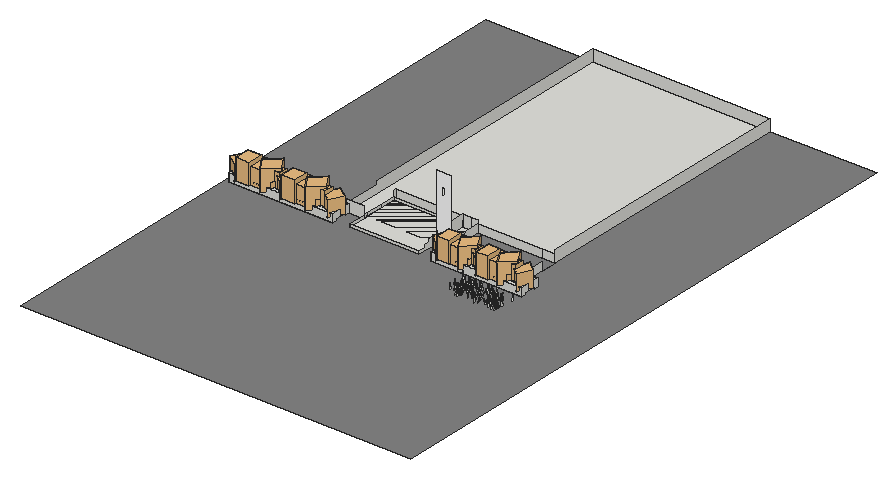
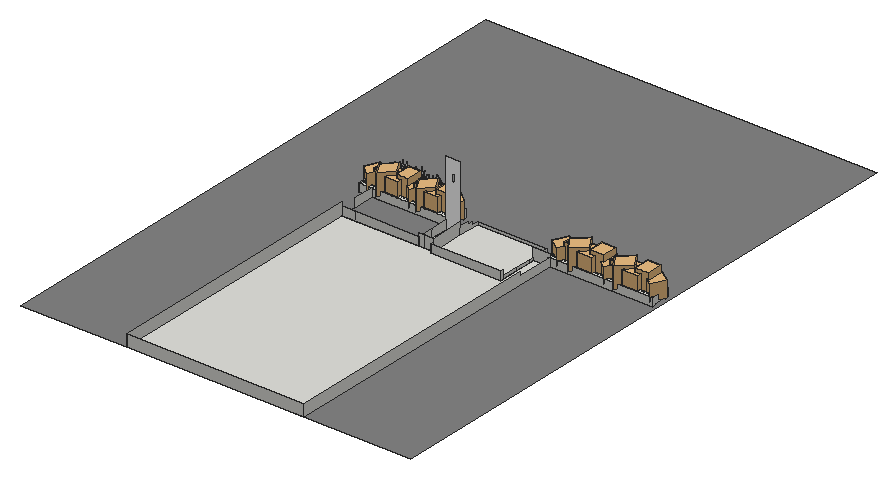
# SketchUp Ruby script. Lengths in inches.
U = 1.inch
M = Sketchup.active_model
def pt(a) = Geom::Point3d.new(a.map { |v| v * U })
def face(e, loops, mat)
  f = e.add_face(loops[0].map { |a| pt(a) })
  loops[1..].each { |l| e.add_face(l.map { |a| pt(a) }).erase! }
  f.material = f.back_material = mat if mat
  f
end
# faces: each face lists its corners as indices into pts; further lists are holes
def faces(e, pts, list, mat = nil) = list.each { |f| face(e, (f[0].is_a?(Array) ? f : [f]).map { |l| l.map { |i| pts[i] } }, mat) }
# xy, xz, yz: faces in a plane at the given z, y or x. An outline is a flat list of corners, or four numbers for a rectangle; further outlines are holes
def ring(l) = l.size == 4 ? [[l[0], l[1]], [l[2], l[1]], [l[2], l[3]], [l[0], l[3]]] : l.each_slice(2).to_a
def flat(e, list, mat, &to3) = list.each { |f| face(e, (f[0].is_a?(Array) ? f : [f]).map { |l| ring(l).map { |u, v| to3.(u, v) } }, mat) }
def xy(e, z, list, mat = nil) = flat(e, list, mat) { |x, y| [x, y, z] }
def xz(e, y, list, mat = nil) = flat(e, list, mat) { |x, z| [x, y, z] }
def yz(e, x, list, mat = nil) = flat(e, list, mat) { |y, z| [x, y, z] }
def lines(e, pts, list) = list.each { |a, b| e.add_line(pt(pts[a]), pt(pts[b])) }
# prism: a flat outline (further loops are holes) pulled along v
def prism(e, loops, v, mat = nil)
  f = face(e, loops, mat); d = Geom::Vector3d.new(v.map { |x| x * U })
  f.pushpull(f.normal.samedirection?(d) ? d.length : -d.length)
end
def box(e, o, s, mat = nil) = prism(e, [[o, [o[0] + s[0], o[1], o[2]], [o[0] + s[0], o[1] + s[1], o[2]], [o[0], o[1] + s[1], o[2]]]], [0, 0, s[2]], mat)
def at(x, y, z, deg = 0) = Geom::Transformation.translation(pt([x, y, z])) * Geom::Transformation.rotation(ORIGIN, Z_AXIS, deg.degrees)
def axes(o, x, y, z) = Geom::Transformation.new([*x, 0, *y, 0, *z, 0, *pt(o).to_a, 1])
def part(name) = M.definitions.add(name)
# library, detail: a bought-in or finely detailed component or shape, given as its bounding box
def library(name, o, s) = part(name).tap { |d| box(d.entities, o, s) }
def detail(e, o, s) = box(e.add_group.entities, o, s)
def put(e, d, t, mat = nil) = e.add_instance(d, t).tap { |i| i.material = mat if mat }
def group(e, t, mat = nil) = e.add_group.tap { |g| g.transformation = t; g.material = mat if mat }.entities
root = M.entities
M.materials.add("Material__1").color = [95, 70, 46]
M.materials.add("[Color M00]").color = [255, 255, 255]
M.materials.add("[Tile Grey]").color = [132, 132, 132]
c1 = part("fur_instance\#9")
p = [[0.8125,0,1.79],[0.67,-0.02,1.48],[0,-0.11,0],[0,0.11,0]]
faces(c1.entities,p,[[0,1,2,3]])
c2 = library("Areca palm plant",[0,0,0],[49.1,36.6,54.46])
c3 = library("Group\#74",[-84.69,-90.07,-0.36],[176.51,175.13,171.4])
c4 = library("Group20\#1",[-20.81,-17.08,3.79],[39.86,39.43,37.51])
c5 = library("Group\#130",[-7.34,-1.2,0],[38.67,35.81,49.04])
c6 = library("Group38\#2",[14.01,28.44,-23.43],[18.58,18.32,38.89])
c7 = part("Group\#69")
put(c7.entities,c2,axes([-6.2,158.41,6.08],[0.45017,-0.56191,0],[0.66137,0.52986,0],[0,0,0.72]))
put(c7.entities,c2,axes([-6.2,56.6,6.08],[0.45017,-0.56191,0],[0.66137,0.52986,0],[0,0,0.72]))
put(c7.entities,c3,axes([14.93,193.18,6.05],[-0.04961,-0.08593,0],[0.08593,-0.04961,0],[0,0,0.10522]))
put(c7.entities,c3,axes([14.93,145.87,6.05],[-0.04961,-0.08593,0],[0.08593,-0.04961,0],[0,0,0.10522]))
put(c7.entities,c3,axes([14.93,173.12,6.05],[-0.04961,-0.08593,0],[0.08593,-0.04961,0],[0,0,0.10522]))
put(c7.entities,c4,axes([18.97,79.98,4.77],[0,0.85,0],[-0.85,0,0],[0,0,0.85]))
put(c7.entities,c5,axes([24.9375,89.91,8],[0,0.79,0],[-0.79,0,0],[0,0,0.79]))
put(c7.entities,c6,axes([-4.1,-1.15,28.17],[0.8848,0,0],[0,0.94674,0],[0,0,0.85826]))
put(c7.entities,c3,axes([14.93,44.05,6.05],[-0.04961,-0.08593,0],[0.08593,-0.04961,0],[0,0,0.10522]))
put(c7.entities,c3,axes([14.93,71.3,6.05],[-0.04961,-0.08593,0],[0.08593,-0.04961,0],[0,0,0.10522]))
put(c7.entities,c3,axes([17.19,121.23,6.07],[-0.08133,-0.14087,0],[0.14087,-0.08133,0],[0,0,0.1725]))
put(c7.entities,c3,axes([14.93,91.37,6.05],[-0.04961,-0.08593,0],[0.08593,-0.04961,0],[0,0,0.10522]))
g1 = group(c7.entities,at(0,0,0))
xy(g1,0,[[0,0,6,234.8],[30,0,36,234.8]])
xy(g1,3,[[6,0,30,234.8]])
xy(g1,7,[[6,5,30,229.8]],"Material__1")
xy(g1,15,[[[0,0,36,234.8],[6,5,30,229.8]]])
xz(g1,0,[[0,0,6,0,6,3,30,3,30,0,36,0,36,15,0,15]])
xz(g1,5,[[6,7,30,15]])
xz(g1,229.8,[[6,7,30,15]])
xz(g1,234.8,[[0,0,0,15,36,15,36,0,30,0,30,3,6,3,6,0]])
yz(g1,0,[[0,0,234.8,15]])
yz(g1,6,[[0,0,234.8,3],[5,7,229.8,15]])
yz(g1,30,[[0,0,234.8,3],[5,7,229.8,15]])
yz(g1,36,[[0,0,234.8,15]])
put(c7.entities,c5,axes([24.9375,191.72,8],[0,0.79,0],[-0.79,0,0],[0,0,0.79]))
put(c7.entities,c6,axes([-4.1,100.66,28.17],[0.8848,0,0],[0,0.94674,0],[0,0,0.85826]))
put(c7.entities,c4,axes([18.97,181.79,4.77],[0,0.85,0],[-0.85,0,0],[0,0,0.85]))
put(c7.entities,c3,axes([17.19,223.04,6.07],[-0.08133,-0.14087,0],[0.14087,-0.08133,0],[0,0,0.1725]))
put(c7.entities,c3,axes([17.19,15.79,6.07],[-0.08133,-0.14087,0],[0.14087,-0.08133,0],[0,0,0.1725]))
xy(root,-21.625,[[226.86,484.17,355.41,484.17,355.41,524.55,382.6,524.55,382.6,585.58,355.41,585.58,355.41,592.02,226.86,592.02],[226.86,484.17,355.41,524.55],[196.6875,516.27,226.86,516.27,226.86,592.02,355.41,592.02,355.41,585.58,525.63,585.58,525.63,1083.4,196.6875,1083.4],[226.86,524.55,355.41,585.58],[355.41,524.55,371.29,585.58],
  [371.29,524.55,382.6,585.58]])
xy(root,-21.625,[[0,5.77,722.32,5.77,722.32,1083.4,525.63,1083.4,525.63,585.58,382.6,585.58,382.6,524.55,355.41,524.55,355.41,484.17,226.86,484.17,226.86,516.27,196.6875,516.27,196.6875,1083.4,0,1083.4]],"[Tile Grey]")
xz(root,484.17,[[226.86,-21.625,355.41,-16.8125]])
xz(root,516.27,[[196.6875,-21.625,226.86,0]])
xz(root,524.55,[[[355.41,-21.625,382.6,100.625],[364.57,61.39,370.5,75.82]]],"[Color M00]")
xz(root,585.58,[[226.86,-21.625,355.41,-16.8125],[355.41,-21.625,371.29,0],[371.29,-21.625,382.6,0],[382.6,-21.625,501.41,-6.4375],[501.41,-21.625,525.63,-6.4375]])
xz(root,592.02,[[226.86,-21.625,355.41,-6.4375]])
xz(root,1083.4,[[196.6875,-21.625,525.63,0]])
yz(root,196.6875,[[516.27,-21.625,516.27,-6.4375,585.58,-6.4375,585.58,0,1083.4,0,1083.4,-21.625]])
yz(root,226.86,[[484.17,-21.625,516.27,-16.8125],[516.27,-21.625,524.55,-16.8125],[524.55,-21.625,555.49,-16.8125],[555.49,-21.625,585.58,-16.8125],[585.58,-21.625,592.02,-6.4375]])
yz(root,355.41,[[484.17,-21.625,524.55,-21.625,524.55,-6.4375,506.86,-6.4375,506.86,-11.5,496.36,-11.5,496.36,-16.8125,484.17,-16.8125],[524.55,-21.625,585.58,0],[585.58,-21.625,592.02,-6.4375]])
yz(root,382.6,[[524.55,-21.625,555.49,-6.4375],[555.49,-21.625,585.58,-6.4375]])
yz(root,525.63,[[512.52,-21.625,555.49,-6.4375],[585.58,-21.625,1083.4,0]])
p = [[525.63,585.58,-21.625],[525.63,555.49,-21.625]]
lines(root,p,[[0,1]])
put(root,c1,axes([474.875,422.99,-21.66],[-2.3678,2.48019,1.72309],[2.76192,2.66404,-0.03926],[1.22155,-1.2159,3.42875]))
put(root,c1,axes([537.98,422.73,-21.66],[-7.39383,1.79038,1.19471],[1.82356,7.48136,0.07416],[1.14343,-0.35412,7.60715]))
put(root,c1,axes([543.77,423.5,-21.66],[2.87262,5.81566,3.24646],[6.49078,-3.23727,0.05584],[-1.49368,-2.88298,6.48619]))
put(root,c1,axes([506.33,423.58,-21.66],[7.01213,2.59998,3.36264],[2.81322,-7.70163,0.08845],[-3.18638,-1.07803,7.47811]))
put(root,c1,axes([470.45,423.2,-21.66],[4.47916,2.33614,0.04477],[2.33654,-4.47877,-0.05982],[-0.01203,-0.07375,5.05142]))
put(root,c1,axes([542.66,424.08,-21.66],[5.19271,0.37939,0.34653],[0.38191,-5.20401,-0.02543],[-0.34375,-0.05067,5.20649]))
put(root,c1,axes([530.99,425.38,-21.66],[1.68942,-4.24341,1.91691],[-4.60334,-1.82876,0.00876],[-0.70022,1.78447,4.56734]))
put(root,c1,axes([511.6,424.82,-21.66],[5.53821,4.98185,1.27941],[5.04776,-5.62536,0.05401],[-0.98782,-0.81487,7.449]))
put(root,c1,axes([491.43,426.85,-21.66],[3.58428,-2.61771,1.24135],[-2.70899,-3.7283,-0.04015],[-1.02701,0.69843,4.43823]))
put(root,c1,axes([544.11,427.84,-21.66],[-2.72992,2.63061,1.69887],[2.87463,2.99911,-0.02472],[1.24209,-1.1593,3.79104]))
put(root,c1,axes([477.83,428.61,-21.66],[-7.83982,-0.95667,1.33619],[-0.96404,7.9519,0.03699],[1.33088,0.12461,7.89789]))
put(root,c1,axes([475.53,428.38,-21.66],[4.582,2.26461,1.64468],[2.3704,-4.81752,0.02956],[-1.48816,-0.70087,5.111]))
put(root,c1,axes([478.9,428.32,-21.66],[6.34041,1.92452,0.88463],[1.94009,-6.39712,0.01179],[-0.84995,-0.24555,6.62604]))
put(root,c1,axes([521.17,429.74,-21.66],[-3.91396,0.19988,0.40503],[0.19284,3.93443,-0.07818],[0.40843,0.05784,3.91828]))
put(root,c1,axes([503.17,430.17,-21.66],[4.73571,-1.08461,0.9225],[-1.0987,-4.82145,-0.02851],[-0.90568,0.17765,4.85824]))
put(root,c1,axes([508.71,430.94,-21.66],[6.16535,-1.94029,0.16764],[-1.94054,-6.16752,-0.01601],[-0.16472,0.03505,6.46343]))
put(root,c1,axes([545.17,431.18,-21.66],[-1.95958,-4.83915,1.26512],[-4.97855,2.01787,0.00704],[0.48156,1.1699,5.22085]))
put(root,c1,axes([473.6875,431.78,-21.66],[3.80262,-6.94068,2.14426],[-7.19034,-3.9408,-0.00453],[-1.0344,1.87826,7.9141]))
put(root,c1,axes([525.47,430.04,-21.66],[4.69542,3.0157,0.91715],[3.05189,-4.76105,0.03053],[-0.78841,-0.46959,5.58037]))
put(root,c1,axes([499.41,433.05,-21.66],[-2.16653,-7.31637,0.90738],[-7.36569,2.18851,0.05952],[0.3151,0.85299,7.63018]))
put(root,c1,axes([523.5,431.74,-21.66],[1.81522,-3.21568,0.8696],[-3.29805,-1.87418,-0.04607],[-0.46866,0.73395,3.69235]))
put(root,c1,axes([495.33,431.29,-21.66],[4.4988,1.24272,1.44893],[1.33102,-4.70119,-0.10058],[-1.36826,-0.48722,4.6662]))
put(root,c1,axes([455.36,431.84,-21.66],[1.09401,4.63876,2.44173],[5.21296,-1.22556,-0.00737],[-0.55243,-2.37843,4.76601]))
put(root,c1,axes([531.0625,432.21,-21.66],[3.86213,1.08614,0.2172],[1.09096,-3.86634,-0.0646],[-0.19154,-0.12107,4.01143]))
put(root,c1,axes([495.47,433.7,-21.66],[-6.50715,-2.26194,0.29712],[-2.26712,6.51165,-0.07913],[0.25462,0.17236,6.88863]))
put(root,c1,axes([529.4375,432.58,-21.66],[2.64561,4.33348,1.24236],[4.47199,-2.70465,-0.08904],[-0.56902,-1.10798,5.07645]))
put(root,c1,axes([522.83,434.75,-21.66],[0.27233,-6.25887,1.87066],[-6.53155,-0.29195,-0.02597],[-0.1084,1.8677,6.26474]))
put(root,c1,axes([469.08,433.68,-21.66],[-5.48361,2.04542,0.49712],[2.0602,5.49974,0.09665],[0.43181,-0.2646,5.85187]))
put(root,c1,axes([524,433.6875,-21.66],[2.95956,2.83712,0.75066],[2.89518,-2.997,-0.08741],[-0.48027,-0.58351,4.09885]))
put(root,c1,axes([461.68,433.21,-21.66],[4.96936,4.425,0.65774],[4.44372,-4.99597,0.03757],[-0.51632,-0.4092,6.65385]))
put(root,c1,axes([461.31,433.36,-21.66],[3.13584,4.70476,0.63652],[4.72939,-3.16238,0.0748],[-0.41563,-0.48786,5.65355]))
put(root,c1,axes([534.39,438.46,-21.66],[-0.28609,-7.90952,0.17476],[-7.91116,0.28452,-0.07401],[-0.06767,0.17732,7.91434]))
put(root,c1,axes([468.52,434.93,-21.66],[-1.71851,4.03919,1.0736],[4.16688,1.74577,0.10182],[0.32374,-1.02868,4.3884]))
put(root,c1,axes([467.48,435.93,-21.66],[-3.40834,-0.81843,0.94444],[-0.85751,3.5273,-0.03792],[0.90911,0.25869,3.50503]))
put(root,c1,axes([528.77,436,-21.66],[6.1687,-0.67373,2.21616],[-0.70194,-6.55164,-0.0379],[-2.20738,0.2006,6.20527]))
put(root,c1,axes([467.7,436.37,-21.66],[-3.21218,-2.63282,1.4726],[-2.81239,3.39173,-0.07071],[1.09119,0.99138,4.15269]))
put(root,c1,axes([460.17,437.6875,-21.66],[-1.26664,-5.03308,1.07763],[-5.14261,1.28411,-0.04714],[0.2163,1.05675,5.1898]))
put(root,c1,axes([507.95,438.18,-21.66],[8.10386,-2.02713,0.06413],[-2.02706,-8.10412,-0.01624],[-0.06615,-0.00019,8.35354]))
put(root,c1,axes([492.31,437.88,-21.66],[-6.58404,0.20466,2.39247],[0.20033,7.00521,-0.04793],[2.39284,-0.02336,6.58705]))
put(root,c1,axes([543.59,440.35,-21.66],[4.25947,-6.86655,0.67935],[-6.89421,-4.26807,0.08653],[-0.2843,0.62304,8.07992]))
put(root,c1,axes([481,437.94,-21.66],[-3.95377,2.90545,0.68572],[2.92437,3.99824,-0.07937],[0.59996,-0.34142,4.90588]))
put(root,c1,axes([473.61,438.64,-21.66],[-3.58743,2.64736,0.43412],[2.66538,3.59954,0.07504],[0.30449,-0.3184,4.45786]))
put(root,c1,axes([477.97,440.8,-21.66],[-6.75441,-2.93713,0.31923],[-2.94167,6.75982,-0.04619],[0.27431,0.1697,7.36523]))
put(root,c1,axes([457.1875,441.18,-21.66],[-4.34525,-4.69158,2.51984],[-5.05188,4.66036,-0.03462],[1.68493,1.87398,6.3946]))
put(root,c1,axes([487.51,441.39,-21.66],[-6.3571,-0.05635,1.63328],[-0.03082,6.56286,0.10646],[1.63396,-0.09544,6.35645]))
put(root,c1,axes([467.11,439.99,-21.66],[4.12664,4.96749,0.53315],[4.97839,-4.14664,0.10195],[-0.41933,-0.34468,6.45715]))
put(root,c1,axes([458.4375,443.28,-21.66],[-1.93771,-4.14246,0.35212],[-4.15628,1.93921,-0.05843],[0.0961,0.34375,4.57288]))
put(root,c1,axes([527.59,442.34,-21.66],[3.42061,-2.16163,2.16053],[-2.46149,-3.8706,0.02453],[-1.81151,1.17767,4.04631]))
put(root,c1,axes([461.96,444.47,-21.66],[-0.71572,-3.67555,0.46048],[-3.70429,0.70984,-0.09154],[-0.00255,0.46948,3.74347]))
put(root,c1,axes([476.59,443.32,-21.66],[-1.48065,3.15767,1.46809],[3.42197,1.61497,-0.02236],[0.64523,-1.31889,3.48751]))
put(root,c1,axes([484.46,445.48,-21.66],[-3.64802,-5.0358,0.07825],[-5.03596,3.64854,0.02575],[0.06676,0.04827,6.21825]))
put(root,c1,axes([481.78,444.82,-21.66],[5.0258,-2.8928,2.35137],[-3.11716,-5.42578,-0.01254],[-2.04464,1.16127,5.79886]))
put(root,c1,axes([473.82,443.9375,-21.66],[1.01663,5.56132,0.68679],[5.60282,-1.02017,-0.03274],[-0.09106,-0.68151,5.65338]))
put(root,c1,axes([493.64,448.68,-21.66],[-0.44109,-6.89492,0.21564],[-6.89758,0.44393,0.08524],[0.09888,0.20974,6.90849]))
put(root,c1,axes([498.125,444.22,-21.66],[1.00933,7.00307,0.82634],[7.04916,-1.02422,0.06983],[-0.18746,-0.80782,7.07509]))
put(root,c1,axes([468.7,448.15,-21.66],[0.77798,-4.23548,0.16889],[-4.23878,-0.77834,0.00619],[-0.02442,0.16723,4.30633]))
put(root,c1,axes([474.21,446.04,-21.66],[-3.97928,1.73175,0.54979],[1.73454,4.01483,-0.09183],[0.54094,-0.13447,4.3388]))
put(root,c1,axes([496.54,447.42,-21.66],[-3.07228,-3.20464,1.70758],[-3.41257,3.31254,0.07678],[1.24093,1.17551,4.43878]))
put(root,c1,axes([528.55,447.74,-21.66],[6.63487,-1.65212,1.91106],[-1.73662,-6.8834,0.0785],[-1.83462,0.54083,6.83702]))
put(root,c1,axes([529.74,447.62,-21.66],[-4.97089,0.8761,1.32855],[0.91857,5.13772,0.0489],[1.29955,-0.28038,5.04727]))
put(root,c1,axes([463.19,448.625,-21.66],[4.72126,-4.87179,1.88096],[-5.03873,-4.91595,-0.08523],[-1.37242,1.28908,6.78361]))
put(root,c1,axes([529.72,446.86,-21.66],[-3.26703,2.9675,0.38966],[2.97957,3.27925,0.00816],[0.28293,-0.26806,4.41355]))
put(root,c1,axes([535.25,449.04,-21.66],[-5.46396,-3.21591,2.3792],[-3.43589,5.83542,-0.00311],[2.04873,1.20967,6.3401]))
put(root,c1,axes([469.13,448.83,-21.66],[-0.34348,3.88251,1.09091],[4.02925,0.37671,-0.07204],[0.17064,-1.07988,3.89701]))
put(root,c1,axes([518.67,450.41,-21.66],[2.48728,-3.44318,0.65298],[-3.47724,-2.52444,-0.0662],[-0.43662,0.49004,4.24707]))
put(root,c1,axes([470.12,450.09,-21.66],[3.33409,-2.8819,1.80128],[-3.12207,-3.59416,0.02846],[-1.34262,1.20116,4.40689]))
put(root,c1,axes([469.6,450.84,-21.66],[-0.47471,-3.8388,0.84095],[-3.92781,0.49062,0.02236],[0.12592,0.83177,3.86797]))
put(root,c1,axes([523.57,451.83,-21.66],[-4.39451,-5.32367,1.29551],[-5.40377,4.48556,0.10243],[0.905,0.93264,6.90237]))
put(root,c1,axes([458.69,449.73,-21.66],[3.76051,3.97563,0.83952],[4.01253,-3.81366,0.08642],[-0.64034,-0.54974,5.47171]))
put(root,c1,axes([513.06,449.95,-21.66],[3.32598,3.77438,0.4675],[3.78797,-3.34308,0.04133],[-0.34022,-0.32329,5.03054]))
put(root,c1,axes([474.84,451.26,-21.66],[4.99939,-0.31235,0.02616],[-0.31267,-4.999,0.06629],[-0.02197,0.06779,5.0087]))
put(root,c1,axes([536.15,451.51,-21.66],[-3.33469,1.40616,1.82105],[1.56398,3.73727,-0.02186],[1.68745,-0.685,3.61897]))
put(root,c1,axes([482.02,449.98,-21.66],[0.04484,6.03011,0.93276],[6.10111,-0.02998,-0.09948],[0.09373,-0.93336,6.02946]))
put(root,c1,axes([479.26,450.5,-21.66],[-0.62472,6.74476,1.37593],[6.88336,0.62526,0.06028],[0.06565,-1.37569,6.77336]))
put(root,c1,axes([531,453.24,-21.66],[1.90593,-3.10212,1.28599],[-3.27722,-2.04084,-0.06594],[-0.73267,1.05893,3.64024]))
put(root,c1,axes([458.91,452.625,-21.66],[3.47844,1.93474,0.04271],[1.93521,-3.47755,-0.07868],[0.00093,-0.08952,3.97952]))
put(root,c1,axes([487.76,454.58,-21.66],[4.25123,5.18566,4.75994],[6.35301,-5.22113,0.01405],[-3.03108,-3.67013,6.70551]))
put(root,c1,axes([501.71,453.04,-21.66],[3.13745,2.7412,0.96065],[2.81213,-3.22064,0.00574],[-0.7273,-0.62763,4.16626]))
put(root,c1,axes([509.96,454.43,-21.66],[-0.91503,4.79321,2.31879],[5.31141,0.98733,0.05504],[0.37492,-2.28894,4.87946]))
put(root,c1,axes([507.33,454.2,-21.66],[3.62939,6.32437,2.66269],[6.74766,-3.83695,-0.08396],[-1.24771,-2.35377,7.2913]))
put(root,c1,axes([471.43,455.21,-21.66],[4.24659,-4.94069,2.32668],[-5.22174,-4.53655,-0.10277],[-1.59916,1.69313,6.51409]))
put(root,c1,axes([491.06,454.63,-21.66],[5.9616,4.7587,3.0284],[5.08757,-6.43918,0.10304],[-2.43578,-1.80245,7.62727]))
put(root,c1,axes([476.54,454.95,-21.66],[-8.26176,0.40654,0.83522],[0.41692,8.30295,0.08258],[0.83009,-0.12394,8.27135]))
put(root,c1,axes([493.94,457.56,-21.66],[-0.46017,-7.01963,1.64197],[-7.20868,0.46604,-0.02793],[0.07879,1.64032,7.03464]))
put(root,c1,axes([505.71,455.17,-21.66],[-4.53452,6.13099,1.20513],[6.2123,4.58336,0.05748],[0.66981,-1.00349,7.62546]))
put(root,c1,axes([460.99,456.91,-21.66],[5.93404,-1.49093,1.99542],[-1.59561,-6.23409,0.08712],[-1.91274,0.57506,6.11785]))
put(root,c1,axes([529.53,456.05,-21.66],[3.18185,3.17768,0.5905],[3.1987,-3.21478,0.06397],[-0.46337,-0.37158,4.49642]))
put(root,c1,axes([478.29,458.73,-21.66],[5.05478,-5.09898,2.04992],[-5.28407,-5.27475,-0.09077],[-1.51011,1.38923,7.17929]))
put(root,c1,axes([493.68,458.48,-21.66],[-3.08604,-1.58363,1.00431],[-1.62158,3.22493,0.10239],[0.94181,0.36349,3.46714]))
put(root,c1,axes([473.125,459.29,-21.66],[3.25628,-4.96201,1.27437],[-5.08219,-3.31911,0.06246],[-0.64574,1.10043,5.93473]))
put(root,c1,axes([488.24,458.97,-21.66],[2.1369,3.02619,1.55246],[3.28055,-2.31782,0.00255],[-0.89775,-1.26656,3.70461]))
put(root,c1,axes([512.12,460.31,-21.66],[-5.21279,-1.15752,0.50027],[-1.17064,5.23306,-0.0898],[0.46875,0.19648,5.33901]))
put(root,c1,axes([510.08,461.57,-21.66],[1.37866,-6.43403,1.32521],[-6.55871,-1.42426,-0.09169],[-0.36909,1.27608,6.57944]))
put(root,c1,axes([516.52,459.55,-21.66],[2.68207,4.86571,0.6841],[4.89534,-2.71316,0.10499],[-0.42283,-0.54794,5.55496]))
put(root,c1,axes([546.71,461.15,-21.66],[-2.11834,3.44874,0.2067],[3.45458,2.11778,0.0692],[0.04913,-0.21236,4.04678]))
put(root,c1,axes([455.26,460.75,-21.66],[-5.44191,5.3364,0.6963],[5.36336,5.45938,0.07682],[0.44311,-0.54257,7.6214]))
put(root,c7,axes([549.33,479.47,-21.625],[0,1,0],[-0.72,0,0],[0,0,1]))
put(root,c7,axes([200.13,479.47,-21.625],[0,1,0],[-0.82597,0,0],[0,0,1]))
